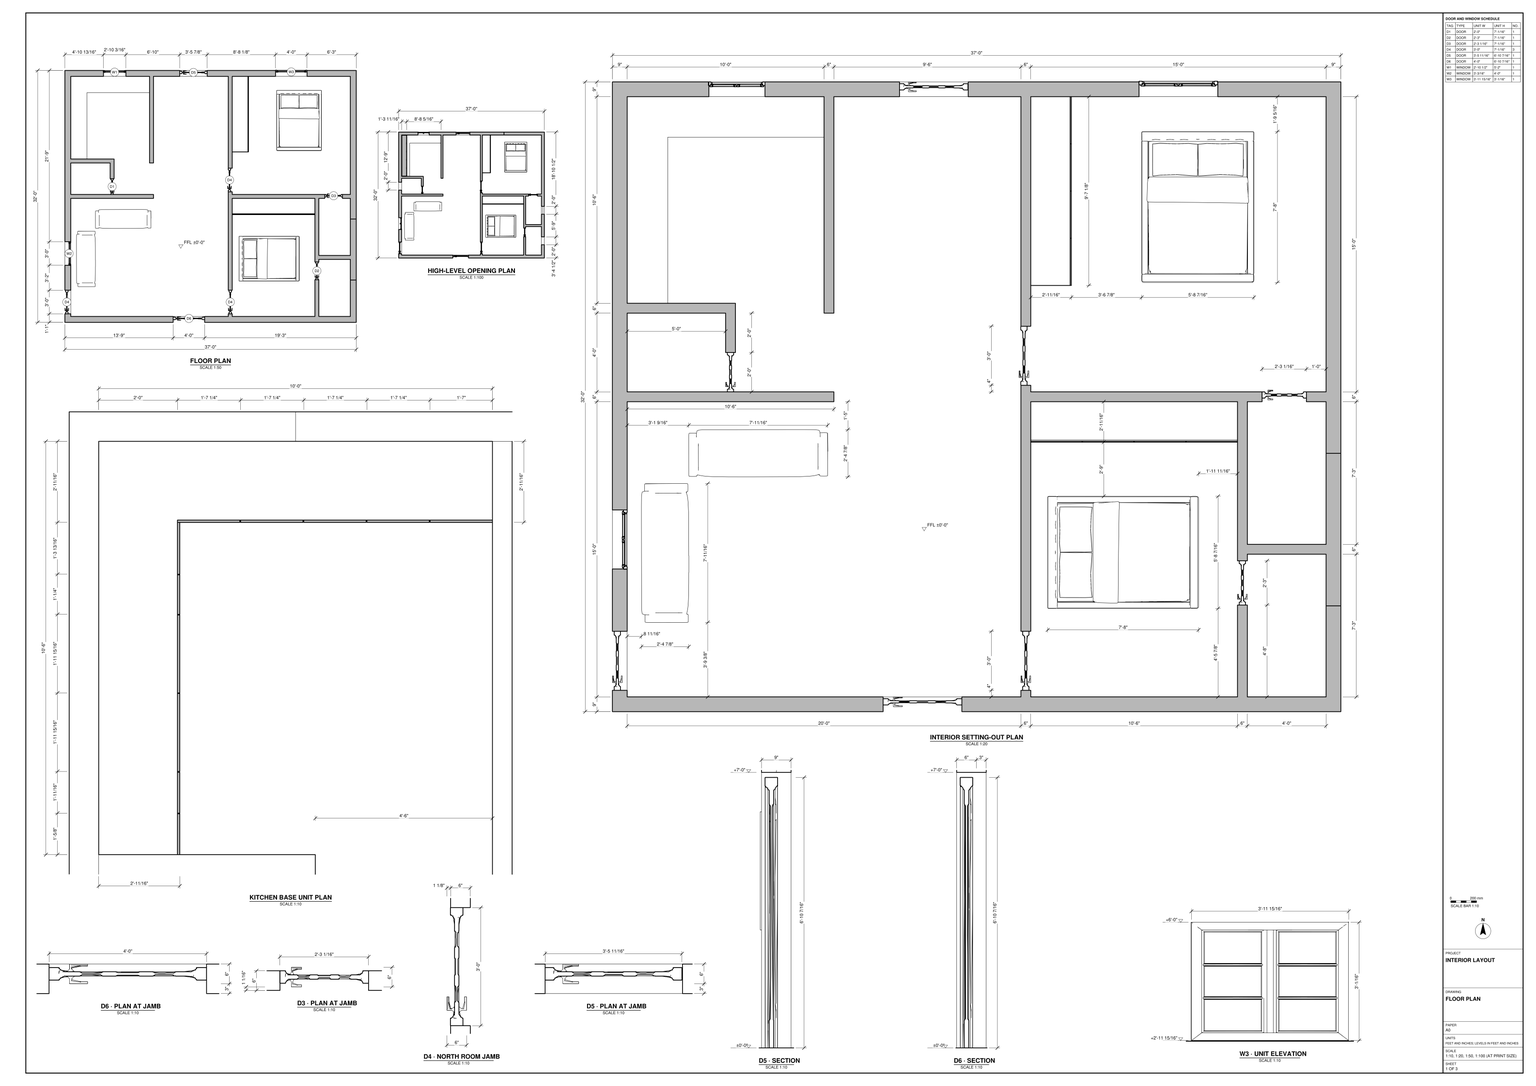
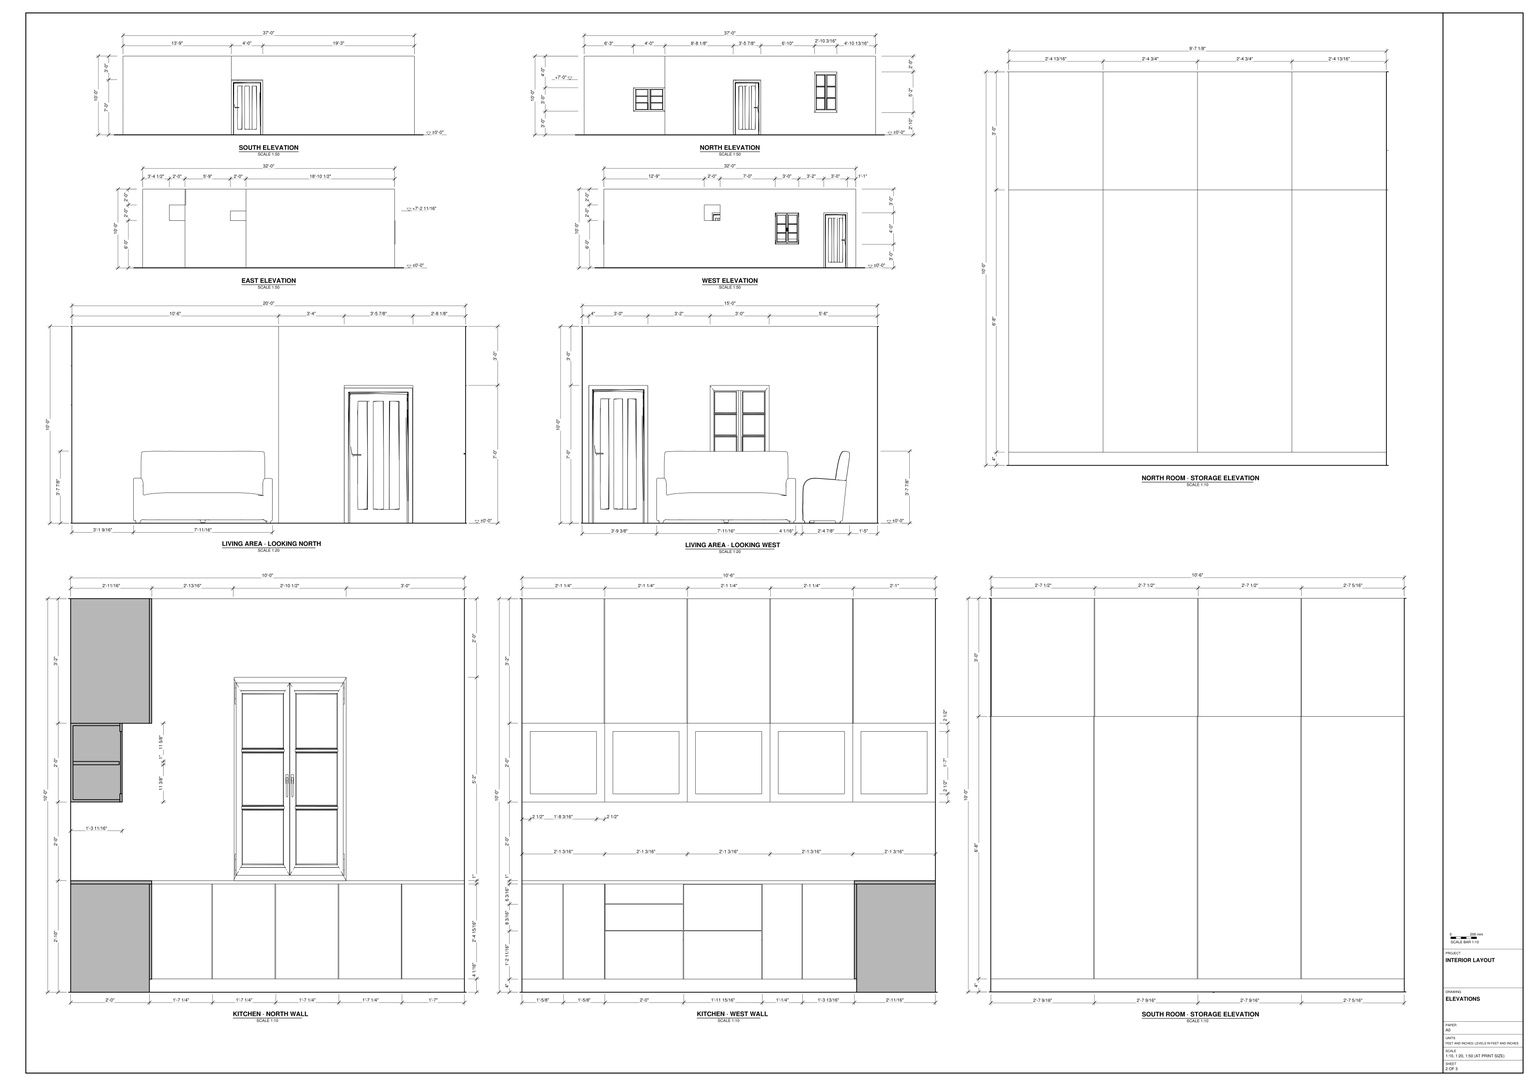
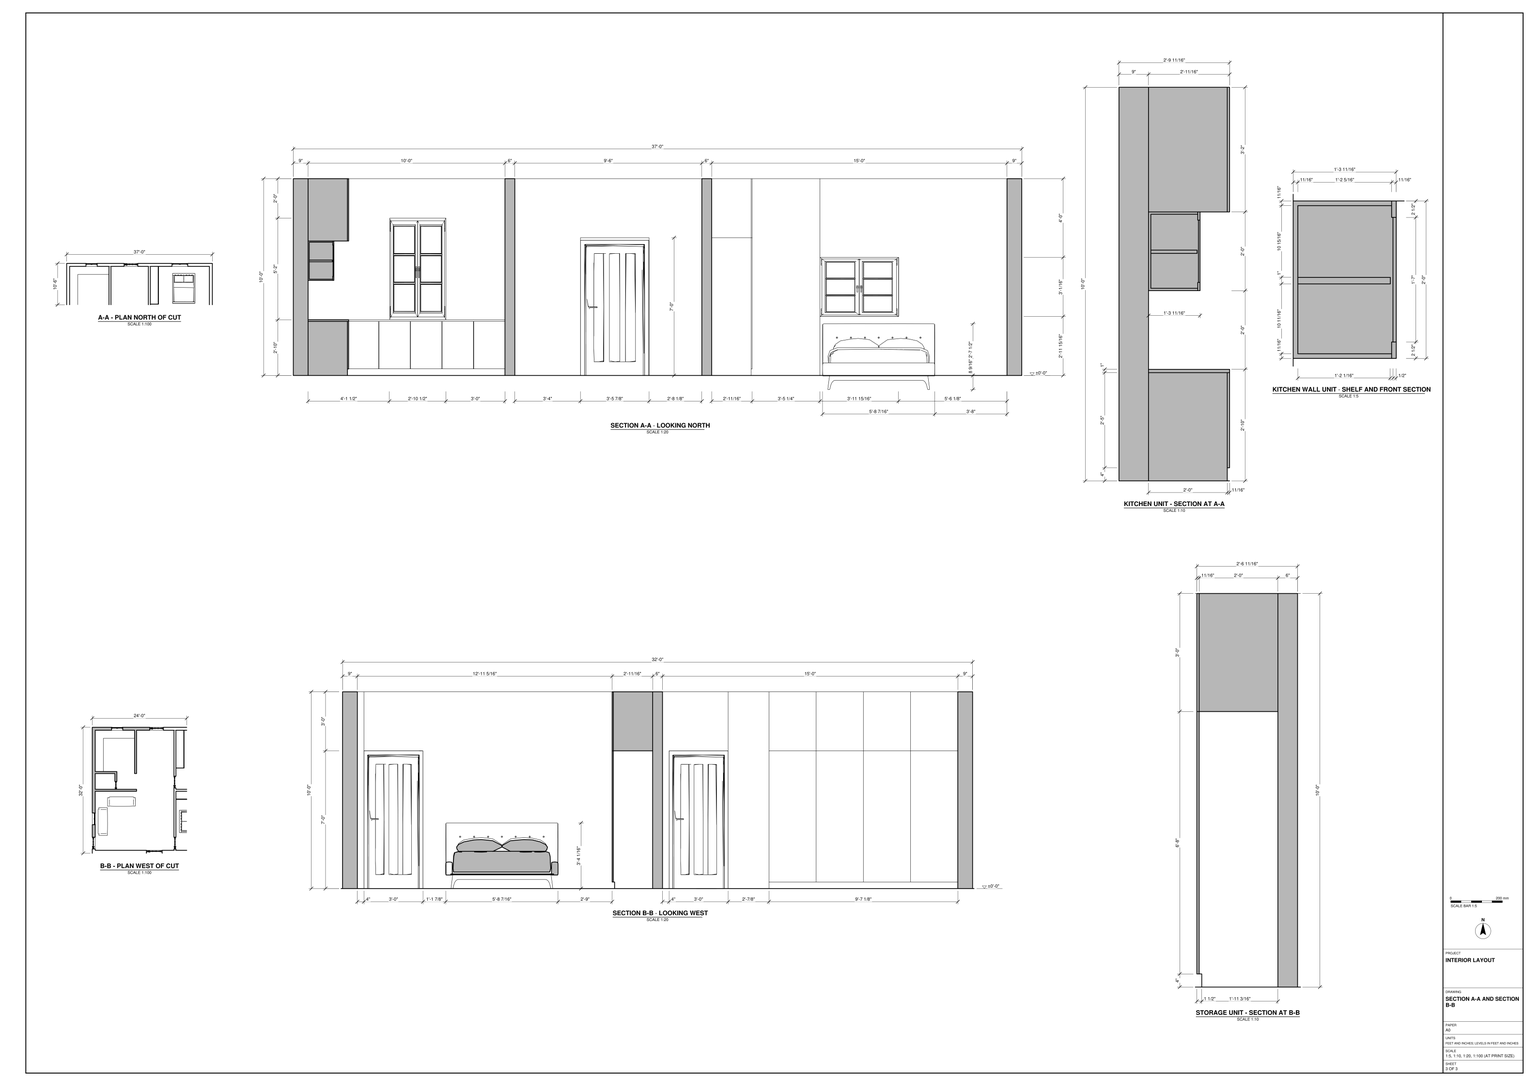
Build the interior in SketchUp from task_files/diagram_01.pdf. Work in feet and inches. The overall model extents are 270'-2 11/16" along X, 182'-10 15/16" along Y and 10'-8 9/16" along Z. These are the full model extents, not the room-setting dimensions. Set out the rectangular shell at 37'-0" by 32'-0", with its single finished floor level at ±0'-0".

Model the floor, the 9" perimeter walls and the 6" interior partitions, following the floor plan for wall returns and door positions. Use the high-level opening plan and elevations to set the heads and sills of the openings. Keep the central passage open between the kitchen and the north bedroom. Place the sofas at right angles in the southwest living area, and orient the platform beds as drawn in the two eastern bedrooms.

Build the L-shaped kitchen along the north and west walls. Use the joinery elevations and sections for the worktop, cabinet fronts, drawers, wall units and shelf. Fit the tall storage along the west wall of the north bedroom and the north wall of the south bedroom, matching the panel divisions and plinths. Decor and loose items may be any suitable library components.

Keep shell elements and each furniture or joinery piece in separate groups or components, and use components for repeated parts. Save one SketchUp model as output_files/interior_with_kitchen_joinery_and_furnished_bedrooms.skp.

# SketchUp Ruby script. Lengths in inches.
U = 1.inch
M = Sketchup.active_model
def pt(a) = Geom::Point3d.new(a.map { |v| v * U })
def face(e, loops, mat)
  f = e.add_face(loops[0].map { |a| pt(a) })
  loops[1..].each { |l| e.add_face(l.map { |a| pt(a) }).erase! }
  f.material = f.back_material = mat if mat
  f
end
# faces: each face lists its corners as indices into pts; further lists are holes
def faces(e, pts, list, mat = nil) = list.each { |f| face(e, (f[0].is_a?(Array) ? f : [f]).map { |l| l.map { |i| pts[i] } }, mat) }
# xy, xz, yz: faces in a plane at the given z, y or x. An outline is a flat list of corners, or four numbers for a rectangle; further outlines are holes
def ring(l) = l.size == 4 ? [[l[0], l[1]], [l[2], l[1]], [l[2], l[3]], [l[0], l[3]]] : l.each_slice(2).to_a
def flat(e, list, mat, &to3) = list.each { |f| face(e, (f[0].is_a?(Array) ? f : [f]).map { |l| ring(l).map { |u, v| to3.(u, v) } }, mat) }
def xy(e, z, list, mat = nil) = flat(e, list, mat) { |x, y| [x, y, z] }
def xz(e, y, list, mat = nil) = flat(e, list, mat) { |x, z| [x, y, z] }
def yz(e, x, list, mat = nil) = flat(e, list, mat) { |y, z| [x, y, z] }
def lines(e, pts, list) = list.each { |a, b| e.add_line(pt(pts[a]), pt(pts[b])) }
# prism: a flat outline (further loops are holes) pulled along v
def prism(e, loops, v, mat = nil)
  f = face(e, loops, mat); d = Geom::Vector3d.new(v.map { |x| x * U })
  f.pushpull(f.normal.samedirection?(d) ? d.length : -d.length)
end
def box(e, o, s, mat = nil) = prism(e, [[o, [o[0] + s[0], o[1], o[2]], [o[0] + s[0], o[1] + s[1], o[2]], [o[0], o[1] + s[1], o[2]]]], [0, 0, s[2]], mat)
def at(x, y, z, deg = 0) = Geom::Transformation.translation(pt([x, y, z])) * Geom::Transformation.rotation(ORIGIN, Z_AXIS, deg.degrees)
def axes(o, x, y, z) = Geom::Transformation.new([*x, 0, *y, 0, *z, 0, *pt(o).to_a, 1])
def part(name) = M.definitions.add(name)
# library, detail: a bought-in or finely detailed component or shape, given as its bounding box
def library(name, o, s) = part(name).tap { |d| box(d.entities, o, s) }
def detail(e, o, s) = box(e.add_group.entities, o, s)
def put(e, d, t, mat = nil) = e.add_instance(d, t).tap { |i| i.material = mat if mat }
def group(e, t, mat = nil) = e.add_group.tap { |g| g.transformation = t; g.material = mat if mat }.entities
root = M.entities
M.materials.add("[Color M00]").color = [255, 255, 255]
M.materials.add("[Marble Carrara Gold Floor Tile]").color = [240, 243, 237]
M.materials.add("[Translucent Glass Gray]").color = [128, 128, 128]
M.materials["[Translucent Glass Gray]"].alpha = 0.5
c1 = library("Door 243 067",[-20.85,-3,0],[41.7,6,82.46])
c2 = library("Window 46-30",[-29.96,-2.6,0],[59.92,5.19,59.84])
c3 = library("Tyler Platform Bed",[-34.22,-45.98,0],[68.44,91.98,40.05])
c4 = library("Sofa 142 022",[-42.35,-14.43,0],[84.7,28.86,43.89])
c5 = part("Group\#5")
box(c5.entities,[0,0,0],[19,0.71,28.9375])
c6 = part("Group\#7")
box(c6.entities,[0,0,0],[0.71,12.45,29])
c7 = part("Group\#11")
box(c7.entities,[0,-11.3125,0],[0.71,23.76,14.66])
c8 = part("Group\#16")
prism(c8.entities,[[[0,0,24],[0,25.2,24],[0,25.2,0],[0,0,0]],[[0,2.5,21.5],[0,2.5,2.5],[0,22.7,2.5],[0,22.7,21.5]]],[0.71,0,0])
g1 = group(c8.entities,at(0.21,2.5,2.5))
box(g1,[0,0,0],[0.5,20.2,19],"[Translucent Glass Gray]")
c9 = part("Group\#20")
box(c9.entities,[0,0,0],[0.71,28.78,36])
c10 = part("Group\#19")
box(c10.entities,[0,0,0],[0.71,28.78,80])
c11 = part("Group\#23")
box(c11.entities,[0,0.2,0],[0.71,25,38])
c12 = part("Group\#25")
box(c12.entities,[0.2,0,-44],[31.3,0.71,80],"[Color M00]")
c13 = part("Group\#26")
box(c13.entities,[0.2,0,0],[31.3,0.71,36],"[Color M00]")
xy(root,0,[[[0,0,3242.6875,2194.9375],[913.6875,459.6875,913.6875,472.6875,922.6875,472.6875,922.6875,508.6875,913.6875,508.6875,913.6875,843.6875,1357.6875,843.6875,1357.6875,459.6875,1126.6875,459.6875,1126.6875,468.6875,1078.6875,468.6875,1078.6875,459.6875]],[913.6875,459.6875,1078.6875,459.6875,1078.6875,468.6875,922.6875,468.6875,922.6875,472.6875,913.6875,472.6875],[1126.6875,459.6875,1357.6875,468.6875],[1162.6875,468.6875,1168.6875,472.6875],[1294.6875,468.6875,1300.6875,524.6875],
  [1348.6875,468.6875,1357.6875,500.1875],[1348.6875,500.1875,1353.1875,524.1875],[1353.1875,500.1875,1357.6875,524.1875],[913.6875,508.6875,922.6875,666.6875],[1162.6875,508.6875,1168.6875,508.6875,1168.6875,648.6875,1294.6875,648.6875,1294.6875,551.6875,1300.6875,551.6875,1300.6875,555.6875,1348.6875,555.6875,1348.6875,561.6875,1300.6875,561.6875,1300.6875,648.6875,1309.6875,648.6875,1309.6875,654.6875,1168.6875,654.6875,1168.6875,658.6875,1162.6875,658.6875],
  [1348.6875,524.1875,1357.6875,593.1875],[1348.6875,593.1875,1353.1875,617.1875],[1353.1875,593.1875,1357.6875,617.1875],[1348.6875,617.1875,1357.6875,617.1875,1357.6875,843.6875,1282.6875,843.6875,1282.6875,834.6875,1348.6875,834.6875],[922.6875,648.6875,1048.6875,654.6875],
  [1336.6875,648.6875,1348.6875,654.6875],[913.6875,666.6875,922.6875,666.6875,922.6875,834.6875,982.6875,834.6875,982.6875,843.6875,913.6875,843.6875],[982.6875,678.6875,988.6875,678.6875,988.6875,708.6875,922.6875,708.6875,922.6875,702.6875,982.6875,702.6875],[1162.6875,694.6875,1168.6875,834.6875],[1042.6875,702.6875,1048.6875,834.6875],
  [922.6875,708.6875,946.6875,708.6875,946.6875,810.6875,1042.6875,810.6875,1042.6875,834.6875,922.6875,834.6875],[1168.6875,719.5625,1192.6875,834.6875],[982.6875,834.6875,1088.6875,843.6875],[1088.6875,834.6875,1130.56,843.6875],[1130.56,834.6875,1234.6875,843.6875],
  [1234.6875,834.6875,1282.6875,839.1875],[1234.6875,839.1875,1282.6875,843.6875]])
xy(root,0,[[922.6875,468.6875,1162.6875,468.6875,1162.6875,472.6875,1168.6875,472.6875,1168.6875,468.6875,1294.6875,468.6875,1294.6875,524.6875,1300.6875,524.6875,1300.6875,468.6875,1348.6875,468.6875,1348.6875,555.6875,1300.6875,555.6875,1300.6875,551.6875,1294.6875,551.6875,1294.6875,624.7,1168.6875,624.7,1168.6875,508.6875,1162.6875,508.6875,1162.6875,658.6875,1168.6875,658.6875,1168.6875,654.6875,1309.6875,654.6875,1309.6875,648.6875,1300.6875,648.6875,1300.6875,561.6875,1348.6875,561.6875,1348.6875,648.6875,1336.6875,648.6875,1336.6875,654.6875,1348.6875,654.6875,1348.6875,834.6875,1192.6875,834.6875,1192.6875,719.5625,1168.6875,719.5625,1168.6875,694.6875,1162.6875,694.6875,1162.6875,834.6875,1048.6875,834.6875,1048.6875,702.6875,1042.6875,702.6875,1042.6875,810.6875,946.6875,810.6875,946.6875,708.6875,988.6875,708.6875,988.6875,678.6875,982.6875,678.6875,982.6875,702.6875,922.6875,702.6875,922.6875,654.6875,1048.6875,654.6875,1048.6875,648.6875,922.6875,648.6875],[1168.6875,624.7,1294.6875,648.6875]],"[Marble Carrara Gold Floor Tile]")
xy(root,34,[[972.5,834.6875,1006.6875,843.6875]])
xy(root,36,[[913.6875,546.6875,922.6875,582.6875]])
xy(root,72,[[913.6875,666.6875,922.6875,690.6875]])
xy(root,84,[[913.6875,472.6875,922.6875,508.6875],[913.6875,546.6875,922.6875,582.6875],[982.6875,654.6875,988.6875,678.6875],[1042.6875,654.6875,1048.6875,702.6875],[1088.6875,834.6875,1130.56,843.6875]])
xy(root,96,[[913.6875,666.6875,922.6875,690.6875],[972.5,834.6875,1006.6875,843.6875]])
xy(root,120,[[[913.6875,459.6875,1078.6875,459.6875,1078.6875,468.6875,922.6875,468.6875,922.6875,648.6875,1048.6875,648.6875,1048.6875,834.6875,1162.6875,834.6875,1162.6875,694.6875,1168.6875,694.6875,1168.6875,834.6875,1234.6875,834.6875,1234.6875,843.6875,913.6875,843.6875],[988.6875,654.6875,988.6875,708.6875,922.6875,708.6875,922.6875,834.6875,1042.6875,834.6875,1042.6875,654.6875],[922.6875,654.6875,982.6875,702.6875]]])
xz(root,459.6875,[[913.6875,0,1078.6875,120]])
xz(root,468.6875,[[922.6875,0,1078.6875,120]])
xz(root,472.6875,[[913.6875,0,922.6875,84]])
xz(root,508.6875,[[913.6875,0,922.6875,84]])
xz(root,546.6875,[[913.6875,36,922.6875,84]])
xz(root,582.6875,[[913.6875,36,922.6875,84]])
xz(root,648.6875,[[922.6875,0,1048.6875,120]])
xz(root,654.6875,[[922.6875,0,922.6875,120,982.6875,120,982.6875,84,988.6875,84,988.6875,120,1042.6875,120,1042.6875,84,1048.6875,84,1048.6875,0]])
xz(root,666.6875,[[913.6875,72,918.1875,96],[918.1875,72,922.6875,96]])
xz(root,678.6875,[[982.6875,0,988.6875,84]])
xz(root,690.6875,[[913.6875,72,922.6875,96]])
xz(root,694.6875,[[1162.6875,0,1168.6875,120]])
xz(root,702.6875,[[922.6875,0,982.6875,120],[1042.6875,0,1048.6875,84]])
xz(root,708.6875,[[922.6875,0,946.6875,120],[946.6875,0,988.6875,120]])
xz(root,834.6875,[[[922.6875,0,1042.6875,120],[972.5,34,1006.6875,96]],[1048.6875,0,1088.6875,0,1088.6875,84,1130.56,84,1130.56,0,1162.6875,0,1162.6875,120,1048.6875,120],[1168.6875,0,1234.6875,120]])
xz(root,843.6875,[[[913.6875,0,913.6875,120,1234.6875,120,1234.6875,0,1130.56,0,1130.56,84,1088.6875,84,1088.6875,0],[972.5,34,1006.6875,96]]])
yz(root,913.6875,[[[459.6875,0,459.6875,120,843.6875,120,843.6875,0,508.6875,0,508.6875,84,472.6875,84,472.6875,0],[546.6875,36,582.6875,84],[666.6875,72,690.6875,96]]])
yz(root,922.6875,[[[468.6875,0,472.6875,0,472.6875,84,508.6875,84,508.6875,0,648.6875,0,648.6875,120,468.6875,120],[546.6875,36,582.6875,84]],[[654.6875,0,702.6875,120],[666.6875,72,690.6875,96]],[708.6875,0,834.6875,58],[708.6875,58,834.6875,82],[708.6875,82,834.6875,120]])
yz(root,972.5,[[834.6875,34,839.1875,96],[839.1875,34,843.6875,96]])
yz(root,982.6875,[[678.6875,0,678.6875,84,654.6875,84,654.6875,120,702.6875,120,702.6875,0]])
yz(root,988.6875,[[678.6875,0,708.6875,0,708.6875,120,654.6875,120,654.6875,84,678.6875,84]])
yz(root,1006.6875,[[834.6875,34,843.6875,96]])
yz(root,1042.6875,[[702.6875,0,702.6875,84,654.6875,84,654.6875,120,810.6875,120,810.6875,0],[810.6875,0,834.6875,120]])
yz(root,1048.6875,[[648.6875,0,654.6875,120],[702.6875,0,834.6875,0,834.6875,120,654.6875,120,654.6875,84,702.6875,84]])
yz(root,1078.6875,[[459.6875,0,468.6875,120]])
yz(root,1088.6875,[[834.6875,0,843.6875,84]])
yz(root,1130.56,[[834.6875,0,843.6875,84]])
yz(root,1162.6875,[[694.6875,0,834.6875,120]])
yz(root,1168.6875,[[694.6875,0,834.6875,120]])
yz(root,1234.6875,[[834.6875,0,839.1875,120],[839.1875,0,843.6875,120]])
p = [[982.6875,839.1875,0],[982.6875,839.1875,34],[918.1875,666.6875,0],[918.1875,666.6875,72],[982.6875,839.1875,96],[982.6875,839.1875,120],
  [918.1875,666.6875,96],[918.1875,666.6875,120]]
lines(root,p,[[0,1],[2,3],[4,5],[6,7]])
put(root,c1,axes([1102.6875,465.68,0],[1.15116,0,0],[0,1,0],[0,0,1]))
put(root,c1,at(1109.54,840.68,0))
put(root,c1,axes([1164.55,676.6875,-0.07],[0,0.86337,0],[-1,0,0],[0,0,1.01942]))
put(root,c1,axes([1165.69,490.6875,0],[0,0.86337,0],[-1,0,0],[0,0,1.01942]))
put(root,c1,axes([1297.69,538.1875,0],[0,0.64752,0],[-1,0,0],[0,0,1.01942]))
put(root,c1,axes([1323.17,652.76,-0.07],[0.64843,0,0],[0,1,0],[0,0,1.01943]))
put(root,c1,axes([916.69,490.6875,0],[0,0.86337,0],[-1,0,0],[0,0,1.01942]))
put(root,c1,axes([985.69,666.6875,0],[0,0.57558,0],[-1,0,0],[0,0,1.01942]))
put(root,c2,axes([1258.59,841.52,35.95],[0.8,0,0],[0,1,0],[0,0,0.60248]))
put(root,c2,axes([989.45,841.1,33.97],[0.57531,0,0],[0,1,0],[0,0,1.03655]))
put(root,c2,axes([920.1,564.61,35.97],[0,-0.60347,0],[1,0,0],[0,0,0.80259]))
put(root,c3,at(1225,556.79,0,90))
put(root,c3,at(1270.49,767.36,-8.53))
put(root,c4,at(1002.57,617.26,0))
put(root,c4,at(945.79,556.42,0,90))
g2 = group(root,at(1126.6875,459.6875,0))
xy(g2,0,[[0,0,0,9,36,9,36,13,42,13,42,9,168,9,168,65,174,65,174,9,222,9,222,64.5,231,64.5,231,0]])
xy(g2,72,[[222,40.5,231,64.5]])
xy(g2,84,[[-48,0,0,9]])
xy(g2,96,[[222,40.5,231,65.5]])
xy(g2,120,[[-48,0,231,0,231,65.5,222,65.5,222,9,174,9,174,65,168,65,168,9,42,9,42,13,36,13,36,9,-48,9]])
xz(g2,0,[[0,0,231,0,231,120,-48,120,-48,84,0,84]])
xz(g2,9,[[0,0,0,84,-48,84,-48,120,36,120,36,0],[42,0,168,120],[174,0,222,120]])
xz(g2,13,[[36,0,42,120]])
xz(g2,40.5,[[222,72,231,96]])
xz(g2,64.5,[[222,0,231,72]])
xz(g2,65,[[168,0,174,120]])
xz(g2,65.5,[[222,96,231,120]])
yz(g2,-48,[[0,84,9,120]])
yz(g2,0,[[0,0,9,84]])
yz(g2,36,[[9,0,13,120]])
yz(g2,42,[[9,0,13,120]])
yz(g2,168,[[9,0,65,120]])
yz(g2,174,[[9,0,65,120]])
yz(g2,222,[[9,0,9,120,65.5,120,65.5,96,40.5,96,40.5,72,64.5,72,64.5,0]])
yz(g2,231,[[0,0,64.5,0,64.5,72,40.5,72,40.5,96,65.5,96,65.5,120,0,120]])
g3 = group(root,at(1162.6875,508.6875,0))
xy(g3,0,[[0,0,0,150,6,150,6,146,147,146,147,140,138,140,138,53,186,53,186,108.5,195,108.5,195,15.5,186,15.5,186,47,138,47,138,43,132,43,132,140,6,140,6,0]])
xy(g3,72,[[186,84.5,190.5,108.5],[190.5,84.5,195,108.5]])
xy(g3,84,[[0,-36,6,0],[132,16,138,43],[0,150,6,186]])
xy(g3,86.6875,[[186,84.5,195,108.5]])
xy(g3,120,[[0,-36,6,-36,6,140,132,140,132,16,138,16,138,47,186,47,186,15.5,195,15.5,195,108.5,186,108.5,186,53,138,53,138,140,147,140,147,146,6,146,6,186,0,186]])
xz(g3,-36,[[0,84,6,120]])
xz(g3,0,[[0,0,6,84]])
xz(g3,15.5,[[186,0,190.5,120],[190.5,0,195,120]])
xz(g3,16,[[132,84,138,120]])
xz(g3,43,[[132,0,138,84]])
xz(g3,47,[[138,0,186,120]])
xz(g3,53,[[138,0,186,120]])
xz(g3,84.5,[[186,72,195,86.6875]])
xz(g3,108.5,[[186,0,195,72],[186,86.6875,195,120]])
xz(g3,140,[[6,0,132,120],[138,0,147,120]])
xz(g3,146,[[6,0,147,120]])
xz(g3,150,[[0,0,6,84]])
xz(g3,186,[[0,84,6,120]])
yz(g3,0,[[0,0,0,84,-36,84,-36,120,186,120,186,84,150,84,150,0]])
yz(g3,6,[[0,0,140,0,140,120,-36,120,-36,84,0,84],[146,0,150,0,150,84,186,84,186,120,146,120]])
yz(g3,132,[[43,0,43,84,16,84,16,120,140,120,140,0]])
yz(g3,138,[[43,0,47,0,47,120,16,120,16,84,43,84],[53,0,140,120]])
yz(g3,147,[[140,0,146,120]])
yz(g3,186,[[15.5,0,47,120],[53,0,53,120,108.5,120,108.5,86.6875,84.5,86.6875,84.5,72,108.5,72,108.5,0]])
yz(g3,195,[[15.5,0,108.5,0,108.5,72,84.5,72,84.5,86.6875,108.5,86.6875,108.5,120,15.5,120]])
g4 = group(root,at(1282.6875,617.1875,0))
xy(g4,0,[[66,0,66,31.5,54,31.5,54,37.5,66,37.5,66,217.5,-48,217.5,-48,226.5,75,226.5,75,0]])
xy(g4,36,[[-48,217.5,0,226.5]])
xy(g4,72,[[-48,217.5,0,226.5]])
xy(g4,84,[[27,31.5,54,37.5]])
xy(g4,120,[[66,0,75,0,75,226.5,-48,226.5,-48,217.5,66,217.5,66,37.5,27,37.5,27,31.5,66,31.5]])
xz(g4,0,[[66,0,70.5,120],[70.5,0,75,120]])
xz(g4,31.5,[[54,0,66,0,66,120,27,120,27,84,54,84]])
xz(g4,37.5,[[54,0,54,84,27,84,27,120,66,120,66,0]])
xz(g4,217.5,[[-48,0,66,0,66,120,-48,120,-48,72,0,72,0,36,-48,36]])
xz(g4,226.5,[[-48,0,-48,36,0,36,0,72,-48,72,-48,120,75,120,75,0]])
yz(g4,-48,[[217.5,0,226.5,36],[217.5,72,226.5,120]])
yz(g4,0,[[217.5,36,226.5,72]])
yz(g4,27,[[31.5,84,37.5,120]])
yz(g4,54,[[31.5,0,37.5,84]])
yz(g4,66,[[0,0,31.5,120],[37.5,0,217.5,120]])
yz(g4,75,[[0,0,226.5,120]])
g5 = group(root,at(922.6875,708.6875,0))
xy(g5,0,[[0,0,0,126,120,126,120,102,24,102,24,0]])
xy(g5,33,[[0,0,24,0,24,102,120,102,120,126,0,126]])
xz(g5,0,[[0,0,24,33]])
xz(g5,102,[[24,0,120,4.0625],[24,4.0625,100.8,33],[100.8,4.0625,120,33]])
xz(g5,126,[[0,0,24,33],[24,0,60,33],[60,0,120,33]])
yz(g5,0,[[0,0,102,33],[102,0,126,33]])
yz(g5,24,[[0,0,102,4],[0,4,12.65,33],[12.65,4,25.29,33],[25.29,4,49.29,15.98],[49.29,4,73.25,15.98],
  [73.25,4,85.29,33],[85.29,4,102,33],[25.29,15.98,49.29,24.49],[49.29,15.98,73.25,33],[25.29,24.49,49.29,33]])
yz(g5,120,[[102,0,126,33]])
p = [[100.8,102,4.0625],[100.8,102,4],[24,73.25,24.49],[24,73.29,24.49]]
lines(g5,p,[[0,1],[2,3]])
put(g5,c5,at(43.25,101.29,4.0625))
put(g5,c5,at(24,101.29,4.0625))
put(g5,c5,at(81.75,101.29,4.0625))
put(g5,c5,at(62.5,101.29,4.0625))
g6 = group(g5,at(24,60.61,21.02))
box(g6,[0,-11.3125,-2.1875],[0.71,23.76,13.97])
put(g5,c5,at(101,101.29,4.0625))
g7 = group(g5,at(24,88.84,4))
box(g7,[0,-3.35,0],[0.71,15.8,29])
g8 = group(g5,at(0,0,33))
prism(g8,[[[24,126,0],[60,126,0],[120,126,0],[120,101.29,0],[24.71,101.29,0],[24.71,0,0],[0,0,0],[0,102,0],[0,126,0]]],[0,0,1])
put(g5,c6,at(24,12.65,4))
put(g5,c6,at(24,0,4))
put(g5,c7,at(24,60.61,4))
g9 = group(g5,at(24,72.84,4))
box(g9,[0,0.41,0],[0.71,12.04,29])
g10 = group(g5,at(24,36.68,27.02))
box(g10,[0,-11.3125,0],[0.71,23.76,5.98])
put(g5,c7,at(24,36.65,4))
g11 = group(g5,at(24,36.68,18.85))
box(g11,[0,-11.3125,0],[0.71,23.76,7.97])
g12 = group(root,at(922.6875,708.6875,58))
g13 = group(g12,at(0,0,0))
xy(g13,0,[[0,0,15,126]])
xy(g13,0.71,[[0.71,0.71,15,125.29]])
xy(g13,23.29,[[0.71,0.71,15,125.29]])
xy(g13,24,[[0,0,15,126]])
xz(g13,0,[[0,0,15,24]])
xz(g13,0.71,[[0.71,0.71,15,23.29]])
xz(g13,125.29,[[0.71,0.71,15,23.29]])
xz(g13,126,[[0,0,15,24]])
yz(g13,0,[[0,0,126,24]])
yz(g13,0.71,[[0.71,0.71,125.29,23.29]])
yz(g13,15,[[[0,0,126,24],[0.71,0.71,125.29,23.29]]])
put(g13,c8,at(15,100.8,0))
put(g13,c8,at(15,25.2,0))
put(g13,c8,at(15,75.6,0))
put(g13,c8,at(15,0,0))
put(g13,c8,at(15,50.4,0))
g14 = group(g12,at(0.71,0.71,11.35))
box(g14,[0,0,0],[14.09,124.58,1],"[Translucent Glass Gray]")
g15 = group(root,at(1168.6875,719.5625,84))
xy(g15,0,[[0,0,24,115.125]])
xy(g15,36,[[0,0,24,115.125]])
xz(g15,0,[[0,0,24,36]])
xz(g15,115.125,[[0,0,24,36]])
yz(g15,0,[[0,0,115.125,36]])
yz(g15,24,[[0,0,86.34,36],[86.34,0,115.125,36]])
put(g15,c9,at(24,0,0))
put(g15,c9,at(24,57.5625,0))
put(g15,c9,at(24,86.34,0))
put(g15,c9,at(24,28.78,0))
g16 = group(root,at(1168.6875,719.5625,0))
xy(g16,0,[[0,0,24,115.125]])
xy(g16,84,[[0,0,24,115.125]])
xz(g16,0,[[0,0,24,84]])
xz(g16,115.125,[[0,0,24,84]])
yz(g16,0,[[0,0,115.125,84]])
yz(g16,24,[[0,0,115.125,4],[[0,4,115.125,84],[0.71,4.71,114.42,83.29]],[0.71,4.71,114.42,83.29]])
put(g16,c10,at(24,28.78,4))
put(g16,c10,at(24,0,4))
put(g16,c10,at(24,57.5625,4))
put(g16,c10,at(24,86.34,4))
g17 = group(root,at(922.6875,708.6875,82))
xy(g17,0,[[0,0,24,126]])
xy(g17,38,[[0,0,24,126]])
xz(g17,0,[[0,0,24,38]])
xz(g17,126,[[0,0,24,38]])
yz(g17,0,[[0,0,126,38]])
yz(g17,24,[[0,0,100.8,38],[100.8,0,126,38]])
put(g17,c11,at(24,100.8,0))
put(g17,c11,at(24,50.3,0))
put(g17,c11,at(24,25.05,0))
put(g17,c11,at(24,75.55,0))
put(g17,c11,at(24,-0.2,0))
g18 = group(root,at(1168.6875,623.99,0))
prism(g18,[[[126,1.5,0],[126,24.7,0],[126,24.7,84],[126,0.71,84],[126,0.71,4],[126,1.5,4]]],[-126,0,0],"[Color M00]")
put(g18,c12,at(62.93,0,48))
put(g18,c12,at(-0.2,0,48))
put(g18,c12,at(31.37,0,48))
put(g18,c12,at(94.5,0,48))
g19 = group(root,at(1168.6875,623.99,84))
xy(g19,0,[[0,0.71,126,24.7]],"[Color M00]")
xy(g19,36,[[0,0.71,126,24.7]],"[Color M00]")
xz(g19,0.71,[[0,0,94.5,36],[94.5,0,126,36]],"[Color M00]")
xz(g19,24.7,[[0,0,126,36]],"[Color M00]")
yz(g19,0,[[0.71,0,24.7,36]],"[Color M00]")
yz(g19,126,[[0.71,0,24.7,36]],"[Color M00]")
put(g19,c13,at(94.5,0,0))
put(g19,c13,at(0,0,0))
put(g19,c13,at(63,0,0))
put(g19,c13,at(31.5,0,0))
